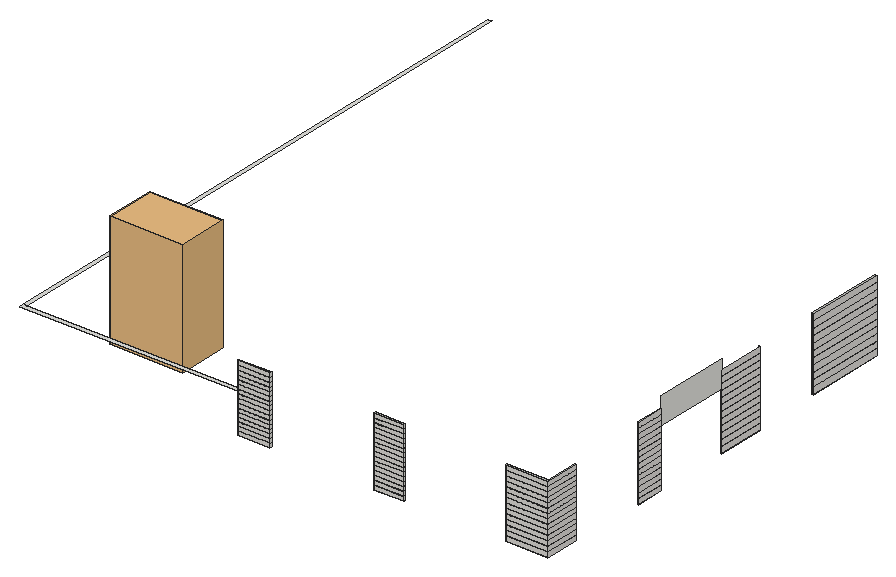
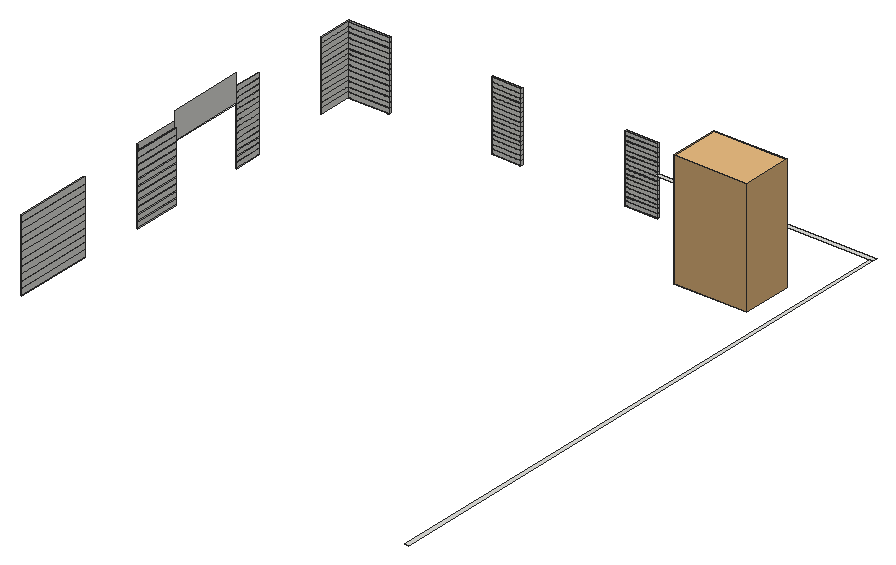
# SketchUp Ruby script. Lengths in inches.
U = 1.inch
M = Sketchup.active_model
def pt(a) = Geom::Point3d.new(a.map { |v| v * U })
def face(e, loops, mat)
  f = e.add_face(loops[0].map { |a| pt(a) })
  loops[1..].each { |l| e.add_face(l.map { |a| pt(a) }).erase! }
  f.material = f.back_material = mat if mat
  f
end
# faces: each face lists its corners as indices into pts; further lists are holes
def faces(e, pts, list, mat = nil) = list.each { |f| face(e, (f[0].is_a?(Array) ? f : [f]).map { |l| l.map { |i| pts[i] } }, mat) }
# xy, xz, yz: faces in a plane at the given z, y or x. An outline is a flat list of corners, or four numbers for a rectangle; further outlines are holes
def ring(l) = l.size == 4 ? [[l[0], l[1]], [l[2], l[1]], [l[2], l[3]], [l[0], l[3]]] : l.each_slice(2).to_a
def flat(e, list, mat, &to3) = list.each { |f| face(e, (f[0].is_a?(Array) ? f : [f]).map { |l| ring(l).map { |u, v| to3.(u, v) } }, mat) }
def xy(e, z, list, mat = nil) = flat(e, list, mat) { |x, y| [x, y, z] }
def xz(e, y, list, mat = nil) = flat(e, list, mat) { |x, z| [x, y, z] }
def yz(e, x, list, mat = nil) = flat(e, list, mat) { |y, z| [x, y, z] }
def lines(e, pts, list) = list.each { |a, b| e.add_line(pt(pts[a]), pt(pts[b])) }
# prism: a flat outline (further loops are holes) pulled along v
def prism(e, loops, v, mat = nil)
  f = face(e, loops, mat); d = Geom::Vector3d.new(v.map { |x| x * U })
  f.pushpull(f.normal.samedirection?(d) ? d.length : -d.length)
end
def box(e, o, s, mat = nil) = prism(e, [[o, [o[0] + s[0], o[1], o[2]], [o[0] + s[0], o[1] + s[1], o[2]], [o[0], o[1] + s[1], o[2]]]], [0, 0, s[2]], mat)
def at(x, y, z, deg = 0) = Geom::Transformation.translation(pt([x, y, z])) * Geom::Transformation.rotation(ORIGIN, Z_AXIS, deg.degrees)
def axes(o, x, y, z) = Geom::Transformation.new([*x, 0, *y, 0, *z, 0, *pt(o).to_a, 1])
def part(name) = M.definitions.add(name)
# library, detail: a bought-in or finely detailed component or shape, given as its bounding box
def library(name, o, s) = part(name).tap { |d| box(d.entities, o, s) }
def detail(e, o, s) = box(e.add_group.entities, o, s)
def put(e, d, t, mat = nil) = e.add_instance(d, t).tap { |i| i.material = mat if mat }
def group(e, t, mat = nil) = e.add_group.tap { |g| g.transformation = t; g.material = mat if mat }.entities
root = M.entities
M.materials.add("[Terrazzo Tile Accent]").color = [224, 221, 217]
c1 = library("tree1",[53.41,58.5,0],[112.17,77.04,177.25])
xy(root,8.42,[[814.625,263.05,816.1875,305.04]])
xy(root,8.5,[[814.625,423.33,816.875,495.84]])
xy(root,9.0625,[[814.625,263.05,816.1875,305.04]])
xy(root,9.44,[[814.625,423.33,816.875,495.84]])
xy(root,11.69,[[547.16,87.66,593.34,90.47]])
xy(root,11.77,[[750.91,87.66,816.1875,87.66,816.1875,140.66,814.625,140.66,814.625,90.47,750.91,90.47]])
xy(root,11.96,[[547.16,87.66,593.34,90.47]])
xy(root,12.4,[[750.91,87.66,750.91,90.47,814.625,90.47,814.625,140.66,816.1875,140.66,816.1875,87.66]])
xy(root,12.86,[[336.5625,87.66,386.78,90.47]])
xy(root,13.19,[[336.5625,87.66,386.78,90.47]])
xy(root,13.92,[[814.625,599,817.6875,719.91]])
xy(root,14.88,[[814.625,599,817.6875,719.91]])
xy(root,16.54,[[814.625,263.05,816.1875,305.04]])
xy(root,17.1875,[[814.625,263.05,816.1875,305.04]])
xy(root,18.43,[[814.625,423.33,816.875,495.84]])
xy(root,18.44,[[547.16,87.66,593.34,90.47]])
xy(root,18.96,[[547.16,87.66,593.34,90.47]])
xy(root,19.26,[[814.625,423.33,816.875,495.84]])
xy(root,19.42,[[336.5625,87.66,386.78,90.47]])
xy(root,19.51,[[336.5625,87.66,386.78,90.47]])
xy(root,19.58,[[750.91,87.66,816.1875,87.66,816.1875,140.66,814.625,140.66,814.625,90.47,750.91,90.47]])
xy(root,20.09,[[750.91,87.66,750.91,90.47,814.625,90.47,814.625,140.66,816.1875,140.66,816.1875,87.66]])
xy(root,24.04,[[814.625,599,817.6875,719.91]])
xy(root,24.67,[[814.625,263.05,816.1875,305.04]])
xy(root,25.01,[[814.625,599,817.6875,719.91]])
xy(root,25.3125,[[814.625,263.05,816.1875,305.04]])
xy(root,25.44,[[547.16,87.66,593.34,90.47]])
xy(root,25.73,[[336.5625,87.66,386.78,90.47]])
xy(root,25.84,[[547.16,87.66,593.34,90.47]])
xy(root,25.88,[[336.5625,87.66,386.78,90.47]])
xy(root,27.27,[[750.91,87.66,816.1875,87.66,816.1875,140.66,814.625,140.66,814.625,90.47,750.91,90.47]])
xy(root,27.71,[[750.91,87.66,750.91,90.47,814.625,90.47,814.625,140.66,816.1875,140.66,816.1875,87.66]])
xy(root,28.25,[[814.625,423.33,816.875,495.84]])
xy(root,28.94,[[814.625,423.33,816.875,495.84]])
xy(root,32.11,[[336.5625,87.66,386.78,90.47]])
xy(root,32.26,[[336.5625,87.66,386.78,90.47]])
xy(root,32.32,[[547.16,87.66,593.34,90.47]])
xy(root,32.4,[[547.16,87.66,593.34,90.47]])
xy(root,32.79,[[814.625,263.05,816.1875,305.04]])
xy(root,33.4375,[[814.625,263.05,816.1875,305.04]])
xy(root,34.17,[[814.625,599,817.6875,719.91]])
xy(root,34.9,[[750.91,87.66,816.1875,87.66,816.1875,140.66,814.625,140.66,814.625,90.47,750.91,90.47]])
xy(root,35.13,[[814.625,599,817.6875,719.91]])
xy(root,35.34,[[750.91,87.66,750.91,90.47,814.625,90.47,814.625,140.66,816.1875,140.66,816.1875,87.66]])
xy(root,37.93,[[814.625,423.33,816.875,495.84]])
xy(root,38.48,[[336.5625,87.66,386.78,90.47]])
xy(root,38.63,[[336.5625,87.66,386.78,90.47],[814.625,423.33,816.875,495.84]])
xy(root,38.88,[[547.16,87.66,593.34,90.47]])
xy(root,38.9,[[547.16,87.66,593.34,90.47]])
xy(root,40.92,[[814.625,263.05,816.1875,305.04]])
xy(root,41.5625,[[814.625,263.05,816.1875,305.04]])
xy(root,42.52,[[750.91,87.66,816.1875,87.66,816.1875,140.66,814.625,140.66,814.625,90.47,750.91,90.47]])
xy(root,42.96,[[750.91,87.66,750.91,90.47,814.625,90.47,814.625,140.66,816.1875,140.66,816.1875,87.66]])
xy(root,44.29,[[814.625,599,817.6875,719.91]])
xy(root,44.86,[[336.5625,87.66,386.78,90.47]])
xy(root,44.94,[[336.5625,87.66,386.78,90.47]])
xy(root,45.26,[[814.625,599,817.6875,719.91]])
xy(root,45.38,[[547.16,87.66,593.34,90.47]])
xy(root,45.46,[[547.16,87.66,593.34,90.47]])
xy(root,47.62,[[814.625,423.33,816.875,495.84]])
xy(root,48.32,[[814.625,423.33,816.875,495.84]])
xy(root,49.04,[[814.625,263.05,816.1875,305.04]])
xy(root,49.6875,[[814.625,263.05,816.1875,305.04]])
xy(root,50.15,[[750.91,87.66,816.1875,87.66,816.1875,140.66,814.625,140.66,814.625,90.47,750.91,90.47]])
xy(root,50.59,[[750.91,87.66,750.91,90.47,814.625,90.47,814.625,140.66,816.1875,140.66,816.1875,87.66]])
xy(root,51.17,[[336.5625,87.66,386.78,90.47]])
xy(root,51.32,[[336.5625,87.66,386.78,90.47]])
xy(root,51.94,[[547.16,87.66,593.34,90.47]])
xy(root,52.03,[[547.16,87.66,593.34,90.47]])
xy(root,54.42,[[814.625,599,817.6875,719.91]])
xy(root,55.38,[[814.625,599,817.6875,719.91]])
xy(root,57.17,[[814.625,263.05,816.1875,305.04]])
xy(root,57.31,[[814.625,423.33,816.875,495.84]])
xy(root,57.54,[[336.5625,87.66,386.78,90.47]])
xy(root,57.77,[[750.91,87.66,816.1875,87.66,816.1875,140.66,814.625,140.66,814.625,90.47,750.91,90.47]])
xy(root,57.8125,[[814.625,263.05,816.1875,305.04]])
xy(root,57.94,[[336.5625,87.66,386.78,90.47]])
xy(root,58.01,[[814.625,423.33,816.875,495.84]])
xy(root,58.15,[[750.91,87.66,750.91,90.47,814.625,90.47,814.625,140.66,816.1875,140.66,816.1875,87.66]])
xy(root,58.5,[[547.16,87.66,593.34,90.47]])
xy(root,58.58,[[547.16,87.66,593.34,90.47]])
xy(root,64.17,[[336.5625,87.66,386.78,90.47]])
xy(root,64.54,[[814.625,599,817.6875,719.91]])
xy(root,64.71,[[336.5625,87.66,386.78,90.47]])
xy(root,65.06,[[547.16,87.66,593.34,90.47]])
xy(root,65.14,[[547.16,87.66,593.34,90.47]])
xy(root,65.29,[[814.625,263.05,816.1875,305.04]])
xy(root,65.33,[[750.91,87.66,816.1875,87.66,816.1875,140.66,814.625,140.66,814.625,90.47,750.91,90.47]])
xy(root,65.51,[[814.625,599,817.6875,719.91]])
xy(root,65.59,[[750.91,87.66,750.91,90.47,814.625,90.47,814.625,140.66,816.1875,140.66,816.1875,87.66]])
xy(root,65.9375,[[814.625,263.05,816.1875,305.04]])
xy(root,67,[[814.625,423.33,816.875,495.84]])
xy(root,67.69,[[814.625,423.33,816.875,495.84]])
xy(root,70.93,[[336.5625,87.66,386.78,90.47]])
xy(root,71.08,[[336.5625,87.66,386.78,90.47]])
xy(root,71.62,[[547.16,87.66,593.34,90.47]])
xy(root,71.77,[[547.16,87.66,593.34,90.47]])
xy(root,72.77,[[750.91,87.66,816.1875,87.66,816.1875,140.66,814.625,140.66,814.625,90.47,750.91,90.47]])
xy(root,73.03,[[750.91,87.66,750.91,90.47,814.625,90.47,814.625,140.66,816.1875,140.66,816.1875,87.66]])
xy(root,73.42,[[814.625,263.05,816.1875,305.04]])
xy(root,74.0625,[[814.625,263.05,816.1875,305.04]])
xy(root,74.67,[[814.625,599,817.6875,719.91]])
xy(root,75.63,[[814.625,599,817.6875,719.91]])
xy(root,76.68,[[814.625,423.33,816.875,495.84]])
xy(root,77.31,[[336.5625,87.66,386.78,90.47]])
xy(root,77.38,[[814.625,423.33,816.875,495.84]])
xy(root,77.52,[[336.5625,87.66,386.78,90.47]])
xy(root,78.25,[[547.16,87.66,593.34,90.47]])
xy(root,78.32,[[547.16,87.66,593.34,90.47]])
xy(root,80.21,[[750.91,87.66,816.1875,87.66,816.1875,140.66,814.625,140.66,814.625,90.47,750.91,90.47]])
xy(root,80.49,[[750.91,87.66,750.91,90.47,814.625,90.47,814.625,140.66,816.1875,140.66,816.1875,87.66]])
xy(root,81.54,[[814.625,263.05,816.1875,305.04]])
xy(root,82.1875,[[814.625,263.05,816.1875,305.04]])
xy(root,83.74,[[336.5625,87.66,386.78,90.47]])
xy(root,84.02,[[336.5625,87.66,386.78,90.47]])
xy(root,84.79,[[814.625,599,817.6875,719.91]])
xy(root,84.8,[[547.16,87.66,593.34,90.47]])
xy(root,84.95,[[547.16,87.66,593.34,90.47]])
xy(root,85.76,[[814.625,599,817.6875,719.91]])
xy(root,86.37,[[814.625,423.33,816.875,495.84]])
xy(root,87.07,[[814.625,423.33,816.875,495.84]])
xy(root,87.67,[[750.91,87.66,816.1875,87.66,816.1875,140.66,814.625,140.66,814.625,90.47,750.91,90.47]])
xy(root,87.99,[[750.91,87.66,750.91,90.47,814.625,90.47,814.625,140.66,816.1875,140.66,816.1875,87.66]])
xy(root,89.67,[[814.625,263.05,816.1875,305.04]])
xy(root,90.24,[[336.5625,87.66,386.78,90.47]])
xy(root,90.3125,[[814.625,263.05,816.1875,305.04]])
xy(root,90.52,[[336.5625,87.66,386.78,90.47]])
xy(root,91.42,[[547.16,87.66,593.34,90.47]])
xy(root,91.57,[[547.16,87.66,593.34,90.47]])
xy(root,94.92,[[814.625,599,817.6875,719.91]])
xy(root,95.17,[[750.91,87.66,816.1875,87.66,816.1875,140.66,814.625,140.66,814.625,90.47,750.91,90.47]])
xy(root,95.43,[[750.91,87.66,750.91,90.47,814.625,90.47,814.625,140.66,816.1875,140.66,816.1875,87.66]])
xy(root,95.88,[[814.625,599,817.6875,719.91]])
xy(root,96.06,[[814.625,423.33,816.875,495.84]])
xy(root,96.74,[[336.5625,87.66,386.78,90.47]])
xy(root,96.76,[[814.625,423.33,816.875,495.84]])
xy(root,96.96,[[336.5625,87.66,386.78,90.47]])
xy(root,97.79,[[814.625,263.05,816.1875,305.04]])
xy(root,98.05,[[547.16,87.66,593.34,90.47]])
xy(root,98.2,[[547.16,87.66,593.34,90.47]])
xy(root,98.4375,[[814.625,263.05,816.1875,305.04],[814.625,305.04,816.1875,423.04],[814.625,423.04,816.1875,423.33]])
xy(root,102.61,[[750.91,87.66,816.1875,87.66,816.1875,140.66,814.625,140.66,814.625,90.47,750.91,90.47]])
xy(root,102.86,[[750.91,87.66,750.91,90.47,814.625,90.47,814.625,140.66,816.1875,140.66,816.1875,87.66]])
xy(root,103.18,[[336.5625,87.66,386.78,90.47]])
xy(root,103.71,[[336.5625,87.66,386.78,90.47]])
xy(root,104.67,[[547.16,87.66,593.34,90.47]])
xy(root,104.88,[[547.16,87.66,593.34,90.47]])
xy(root,105.04,[[814.625,599,817.6875,719.91]])
xy(root,105.75,[[814.625,423.33,816.875,495.84]])
xy(root,105.92,[[814.625,263.05,816.1875,305.04]])
xy(root,106.01,[[814.625,599,817.6875,719.91]])
xy(root,106.44,[[814.625,423.33,816.875,495.84]])
xy(root,106.5625,[[814.625,263.05,816.1875,305.04]])
xy(root,109.93,[[336.5625,87.66,386.78,90.47]])
xy(root,110.05,[[750.91,87.66,816.1875,87.66,816.1875,140.66,814.625,140.66,814.625,90.47,750.91,90.47]])
xy(root,110.36,[[750.91,87.66,750.91,90.47,814.625,90.47,814.625,140.66,816.1875,140.66,816.1875,87.66]])
xy(root,110.46,[[336.5625,87.66,386.78,90.47]])
xy(root,111.36,[[547.16,87.66,593.34,90.47]])
xy(root,111.7,[[547.16,87.66,593.34,90.47]])
xy(root,114.04,[[814.625,263.05,816.1875,305.04]])
xy(root,114.6875,[[814.625,263.05,816.1875,305.04]])
xy(root,115.17,[[814.625,599,817.6875,719.91]])
xy(root,115.43,[[814.625,423.33,816.875,495.84]])
xy(root,116.13,[[814.625,423.33,816.875,495.84],[814.625,599,817.6875,719.91]])
xz(root,87.66,[[547.16,11.96,593.34,18.44],[750.91,12.4,816.1875,19.58],[336.5625,13.19,386.78,19.42],[547.16,18.96,593.34,25.44],[336.5625,19.51,386.78,25.73],
  [750.91,20.09,816.1875,27.27],[547.16,25.84,593.34,32.32],[336.5625,25.88,386.78,32.11],[750.91,27.71,816.1875,34.9],[336.5625,32.26,386.78,38.48],
  [547.16,32.4,593.34,38.88],[750.91,35.34,816.1875,42.52],[336.5625,38.63,386.78,44.86],[547.16,38.9,593.34,45.38],[750.91,42.96,816.1875,50.15],
  [336.5625,44.94,386.78,51.17],[547.16,45.46,593.34,51.94],[750.91,50.59,816.1875,57.77],[336.5625,51.32,386.78,57.54],[547.16,52.03,593.34,58.5],
  [336.5625,57.94,386.78,64.17],[750.91,58.15,816.1875,65.33],[547.16,58.58,593.34,65.06],[336.5625,64.71,386.78,70.93],[547.16,65.14,593.34,71.62],
  [750.91,65.59,816.1875,72.77],[336.5625,71.08,386.78,77.31],[547.16,71.77,593.34,78.25],[750.91,73.03,816.1875,80.21],[336.5625,77.52,386.78,83.74],
  [547.16,78.32,593.34,84.8],[750.91,80.49,816.1875,87.67],[336.5625,84.02,386.78,90.24],[547.16,84.95,593.34,91.42],[750.91,87.99,816.1875,95.17],
  [336.5625,90.52,386.78,96.74],[547.16,91.57,593.34,98.05],[750.91,95.43,816.1875,102.61],[336.5625,96.96,386.78,103.18],[547.16,98.2,593.34,104.67],
  [750.91,102.86,816.1875,110.05],[336.5625,103.71,386.78,109.93],[547.16,104.88,593.34,111.36],[750.91,110.36,816.1875,117.55],[336.5625,110.46,386.78,116.68],
  [547.16,111.7,593.34,118.17]],"[Terrazzo Tile Accent]")
xz(root,90.47,[[547.16,11.69,593.34,11.96],[750.91,11.77,814.625,12.4],[547.16,11.96,593.34,18.44],[750.91,12.4,814.625,19.58],[336.5625,12.86,386.78,13.19],
  [336.5625,13.19,386.78,19.42],[547.16,18.44,593.34,18.96],[547.16,18.96,593.34,25.44],[336.5625,19.42,386.78,19.51],[336.5625,19.51,386.78,25.73],
  [750.91,19.58,814.625,20.09],[750.91,20.09,814.625,27.27],[547.16,25.44,593.34,25.84],[336.5625,25.73,386.78,25.88],[547.16,25.84,593.34,32.32],
  [336.5625,25.88,386.78,32.11],[750.91,27.27,814.625,27.71],[750.91,27.71,814.625,34.9],[336.5625,32.11,386.78,32.26],[336.5625,32.26,386.78,38.48],
  [547.16,32.32,593.34,32.4],[547.16,32.4,593.34,38.88],[750.91,34.9,814.625,35.34],[750.91,35.34,814.625,42.52],[336.5625,38.48,386.78,38.63],
  [336.5625,38.63,386.78,44.86],[547.16,38.88,593.34,38.9],[547.16,38.9,593.34,45.38],[750.91,42.52,814.625,42.96],[750.91,42.96,814.625,50.15],
  [336.5625,44.86,386.78,44.94],[336.5625,44.94,386.78,51.17],[547.16,45.38,593.34,45.46],[547.16,45.46,593.34,51.94],[750.91,50.15,814.625,50.59],
  [750.91,50.59,814.625,57.77],[336.5625,51.17,386.78,51.32],[336.5625,51.32,386.78,57.54],[547.16,51.94,593.34,52.03],[547.16,52.03,593.34,58.5],
  [336.5625,57.54,386.78,57.94],[750.91,57.77,814.625,58.15],[336.5625,57.94,386.78,64.17],[750.91,58.15,814.625,65.33],[547.16,58.5,593.34,58.58],
  [547.16,58.58,593.34,65.06],[336.5625,64.17,386.78,64.71],[336.5625,64.71,386.78,70.93],[547.16,65.06,593.34,65.14],[547.16,65.14,593.34,71.62],
  [750.91,65.33,814.625,65.59],[750.91,65.59,814.625,72.77],[336.5625,70.93,386.78,71.08],[336.5625,71.08,386.78,77.31],[547.16,71.62,593.34,71.77],
  [547.16,71.77,593.34,78.25],[750.91,72.77,814.625,73.03],[750.91,73.03,814.625,80.21],[336.5625,77.31,386.78,77.52],[336.5625,77.52,386.78,83.74],
  [547.16,78.25,593.34,78.32],[547.16,78.32,593.34,84.8],[750.91,80.21,814.625,80.49],[750.91,80.49,814.625,87.67],[336.5625,83.74,386.78,84.02],
  [336.5625,84.02,386.78,90.24],[547.16,84.8,593.34,84.95],[547.16,84.95,593.34,91.42],[750.91,87.67,814.625,87.99],[750.91,87.99,814.625,95.17],
  [336.5625,90.24,386.78,90.52],[336.5625,90.52,386.78,96.74],[547.16,91.42,593.34,91.57],[547.16,91.57,593.34,98.05],[750.91,95.17,814.625,95.43],
  [750.91,95.43,814.625,102.61],[336.5625,96.74,386.78,96.96],[336.5625,96.96,386.78,103.18],[547.16,98.05,593.34,98.2],[547.16,98.2,593.34,104.67],
  [750.91,102.61,814.625,102.86],[750.91,102.86,814.625,110.05],[336.5625,103.18,386.78,103.71],[336.5625,103.71,386.78,109.93],[547.16,104.67,593.34,104.88],
  [547.16,104.88,593.34,111.36],[336.5625,109.93,386.78,110.46],[750.91,110.05,814.625,110.36],[750.91,110.36,814.625,117.55],[336.5625,110.46,386.78,116.68],
  [547.16,111.36,593.34,111.7],[547.16,111.7,593.34,118.17]])
xz(root,140.66,[[814.625,12.4,816.1875,19.58],[814.625,20.09,816.1875,27.27],[814.625,27.71,816.1875,34.9],[814.625,35.34,816.1875,42.52],[814.625,42.96,816.1875,50.15],
  [814.625,50.59,816.1875,57.77],[814.625,58.15,816.1875,65.33],[814.625,65.59,816.1875,72.77],[814.625,73.03,816.1875,80.21],[814.625,80.49,816.1875,87.67],
  [814.625,87.99,816.1875,95.17],[814.625,95.43,816.1875,102.61],[814.625,102.86,816.1875,110.05],[814.625,110.36,816.1875,117.55]])
xz(root,263.05,[[814.625,9.0625,816.1875,16.54],[814.625,17.1875,816.1875,24.67],[814.625,25.3125,816.1875,32.79],[814.625,33.4375,816.1875,40.92],[814.625,41.5625,816.1875,49.04],
  [814.625,49.6875,816.1875,57.17],[814.625,57.8125,816.1875,65.29],[814.625,65.9375,816.1875,73.42],[814.625,74.0625,816.1875,81.54],[814.625,82.1875,816.1875,89.67],
  [814.625,90.3125,816.1875,97.79],[814.625,98.4375,816.1875,105.92],[814.625,106.5625,816.1875,114.04],[814.625,114.6875,816.1875,122.17]])
xz(root,305.04,[[814.625,9.0625,816.1875,16.54],[814.625,17.1875,816.1875,24.67],[814.625,25.3125,816.1875,32.79],[814.625,33.4375,816.1875,40.92],[814.625,41.5625,816.1875,49.04],
  [814.625,49.6875,816.1875,57.17],[814.625,57.8125,816.1875,65.29],[814.625,65.9375,816.1875,73.42],[814.625,74.0625,816.1875,81.54],[814.625,82.1875,816.1875,89.67],
  [814.625,90.3125,816.1875,97.79],[814.625,98.4375,816.1875,105.92],[814.625,105.92,816.1875,106.5625],[814.625,106.5625,816.1875,114.04],[814.625,114.04,816.1875,114.6875],
  [814.625,114.6875,816.1875,122.17]])
xz(root,423.33,[[814.625,9.44,816.875,18.43],[814.625,19.26,816.875,28.25],[814.625,28.94,816.875,37.93],[814.625,38.63,816.875,47.62],[814.625,48.32,816.875,57.31],
  [814.625,58.01,816.875,67],[814.625,67.69,816.875,76.68],[814.625,77.38,816.875,86.37],[814.625,87.07,816.875,96.06],[814.625,96.76,816.875,96.76,816.875,105.75,816.1875,105.75,816.1875,98.4375,814.625,98.4375],
  [814.625,98.4375,816.1875,105.75],[814.625,105.75,816.1875,106.44],[814.625,106.44,816.1875,115.43],[816.1875,106.44,816.875,115.43],[814.625,115.43,816.1875,116.13],
  [816.1875,116.13,816.875,125.12]])
xz(root,495.84,[[814.625,19.26,816.875,28.25],[814.625,28.94,816.875,37.93],[814.625,38.63,816.875,47.62],[814.625,48.32,816.875,57.31],[814.625,58.01,816.875,67],
  [814.625,67.69,816.875,76.68],[814.625,77.38,816.875,86.37],[814.625,87.07,816.875,96.06],[814.625,96.76,816.875,105.75],[814.625,106.44,816.875,115.43],
  [814.625,116.13,816.875,125.12]])
xz(root,599,[[814.625,14.88,817.6875,24.04],[814.625,25.01,817.6875,34.17],[814.625,35.13,817.6875,44.29],[814.625,45.26,817.6875,54.42],[814.625,55.38,817.6875,64.54],
  [814.625,65.51,817.6875,74.67],[814.625,75.63,817.6875,84.79],[814.625,85.76,817.6875,94.92],[814.625,95.88,817.6875,105.04],[814.625,106.01,817.6875,115.17],
  [814.625,116.13,817.6875,125.29]])
xz(root,719.91,[[814.625,14.88,817.6875,24.04],[814.625,25.01,817.6875,34.17],[814.625,35.13,817.6875,44.29],[814.625,45.26,817.6875,54.42],[814.625,55.38,817.6875,64.54],
  [814.625,65.51,817.6875,74.67],[814.625,75.63,817.6875,84.79],[814.625,85.76,817.6875,94.92],[814.625,95.88,817.6875,105.04],[814.625,106.01,817.6875,115.17],
  [814.625,116.13,817.6875,125.29]])
yz(root,336.5625,[[87.66,13.19,90.47,19.42],[87.66,19.51,90.47,25.73],[87.66,25.88,90.47,32.11],[87.66,32.26,90.47,38.48],[87.66,38.63,90.47,44.86],
  [87.66,44.94,90.47,51.17],[87.66,51.32,90.47,57.54],[87.66,57.94,90.47,64.17],[87.66,64.71,90.47,70.93],[87.66,71.08,90.47,77.31],
  [87.66,77.52,90.47,83.74],[87.66,84.02,90.47,90.24],[87.66,90.52,90.47,96.74],[87.66,96.96,90.47,103.18],[87.66,103.71,90.47,109.93],
  [87.66,110.46,90.47,116.68]])
yz(root,386.78,[[87.66,13.19,90.47,19.42],[87.66,19.51,90.47,25.73],[87.66,25.88,90.47,32.11],[87.66,32.26,90.47,38.48],[87.66,38.63,90.47,44.86],
  [87.66,44.94,90.47,51.17],[87.66,51.32,90.47,57.54],[87.66,57.94,90.47,64.17],[87.66,64.71,90.47,70.93],[87.66,71.08,90.47,77.31],
  [87.66,77.52,90.47,83.74],[87.66,84.02,90.47,90.24],[87.66,90.52,90.47,96.74],[87.66,96.96,90.47,103.18],[87.66,103.71,90.47,109.93],
  [87.66,110.46,90.47,116.68]])
yz(root,547.16,[[87.66,11.96,90.47,18.44],[87.66,18.96,90.47,25.44],[87.66,25.84,90.47,32.32],[87.66,32.4,90.47,38.88],[87.66,38.9,90.47,45.38],
  [87.66,45.46,90.47,51.94],[87.66,52.03,90.47,58.5],[87.66,58.58,90.47,65.06],[87.66,65.14,90.47,71.62],[87.66,71.77,90.47,78.25],
  [87.66,78.32,90.47,84.8],[87.66,84.95,90.47,91.42],[87.66,91.57,90.47,98.05],[87.66,98.2,90.47,104.67],[87.66,104.88,90.47,111.36],
  [87.66,111.7,90.47,118.17]])
yz(root,593.34,[[87.66,11.96,90.47,18.44],[87.66,18.96,90.47,25.44],[87.66,25.84,90.47,32.32],[87.66,32.4,90.47,38.88],[87.66,38.9,90.47,45.38],
  [87.66,45.46,90.47,51.94],[87.66,52.03,90.47,58.5],[87.66,58.58,90.47,65.06],[87.66,65.14,90.47,71.62],[87.66,71.77,90.47,78.25],
  [87.66,78.32,90.47,84.8],[87.66,84.95,90.47,91.42],[87.66,91.57,90.47,98.05],[87.66,98.2,90.47,104.67],[87.66,104.88,90.47,111.36],
  [87.66,111.7,90.47,118.17]])
yz(root,750.91,[[87.66,12.4,90.47,19.58],[87.66,20.09,90.47,27.27],[87.66,27.71,90.47,34.9],[87.66,35.34,90.47,42.52],[87.66,42.96,90.47,50.15],
  [87.66,50.59,90.47,57.77],[87.66,58.15,90.47,65.33],[87.66,65.59,90.47,72.77],[87.66,73.03,90.47,80.21],[87.66,80.49,90.47,87.67],
  [87.66,87.99,90.47,95.17],[87.66,95.43,90.47,102.61],[87.66,102.86,90.47,110.05],[87.66,110.36,90.47,117.55]])
yz(root,814.625,[[263.05,8.42,305.04,9.0625],[423.33,8.5,495.84,9.44],[263.05,9.0625,305.04,16.54],[423.33,9.44,495.84,18.43],[90.47,12.4,140.66,19.58],
  [599,14.88,719.91,24.04],[263.05,16.54,305.04,17.1875],[263.05,17.1875,305.04,24.67],[423.33,18.43,495.84,19.26],[423.33,19.26,495.84,28.25],
  [90.47,20.09,140.66,27.27],[263.05,24.67,305.04,25.3125],[599,25.01,719.91,34.17],[263.05,25.3125,305.04,32.79],[90.47,27.71,140.66,34.9],
  [423.33,28.25,495.84,28.94],[423.33,28.94,495.84,37.93],[263.05,32.79,305.04,33.4375],[263.05,33.4375,305.04,40.92],[599,35.13,719.91,44.29],
  [90.47,35.34,140.66,42.52],[423.33,37.93,495.84,38.63],[423.33,38.63,495.84,47.62],[263.05,40.92,305.04,41.5625],[263.05,41.5625,305.04,49.04],
  [90.47,42.96,140.66,50.15],[599,45.26,719.91,54.42],[423.33,47.62,495.84,48.32],[423.33,48.32,495.84,57.31],[263.05,49.04,305.04,49.6875],
  [263.05,49.6875,305.04,57.17],[90.47,50.59,140.66,57.77],[599,55.38,719.91,64.54],[263.05,57.17,305.04,57.8125],[423.33,57.31,495.84,58.01],
  [263.05,57.8125,305.04,65.29],[423.33,58.01,495.84,67],[90.47,58.15,140.66,65.33],[263.05,65.29,305.04,65.9375],[599,65.51,719.91,74.67],
  [90.47,65.59,140.66,72.77],[263.05,65.9375,305.04,73.42],[423.33,67,495.84,67.69],[423.33,67.69,495.84,76.68],[90.47,73.03,140.66,80.21],
  [263.05,73.42,305.04,74.0625],[263.05,74.0625,305.04,81.54],[599,75.63,719.91,84.79],[423.33,76.68,495.84,77.38],[423.33,77.38,495.84,86.37],
  [90.47,80.49,140.66,87.67],[263.05,81.54,305.04,82.1875],[263.05,82.1875,305.04,89.67],[599,85.76,719.91,94.92],[423.33,86.37,495.84,87.07],
  [423.33,87.07,495.84,96.06],[90.47,87.99,140.66,95.17],[263.05,89.67,305.04,90.3125],[263.05,90.3125,305.04,97.79],[90.47,95.43,140.66,102.61],
  [599,95.88,719.91,105.04],[423.33,96.06,495.84,96.76],[423.33,96.76,495.84,105.75],[263.05,97.79,305.04,98.4375],[263.05,98.4375,305.04,105.92],
  [90.47,102.86,140.66,110.05],[423.33,105.75,495.84,106.44],[263.05,105.92,305.04,106.5625],[599,106.01,719.91,115.17],[423.33,106.44,495.84,115.43],
  [263.05,106.5625,305.04,114.04],[90.47,110.36,140.66,117.55],[263.05,114.04,305.04,114.6875],[263.05,114.6875,305.04,122.17],[423.33,115.43,495.84,116.13],
  [599,116.13,719.91,125.29]])
yz(root,816.1875,[[305.04,98.4375,423.33,140.0625]])
yz(root,816.1875,[[263.05,9.0625,305.04,16.54],[87.66,12.4,140.66,19.58],[263.05,17.1875,305.04,24.67],[87.66,20.09,140.66,27.27],[263.05,25.3125,305.04,32.79],
  [87.66,27.71,140.66,34.9],[263.05,33.4375,305.04,40.92],[87.66,35.34,140.66,42.52],[263.05,41.5625,305.04,49.04],[87.66,42.96,140.66,50.15],
  [263.05,49.6875,305.04,57.17],[87.66,50.59,140.66,57.77],[263.05,57.8125,305.04,65.29],[87.66,58.15,140.66,65.33],[87.66,65.59,140.66,72.77],
  [263.05,65.9375,305.04,73.42],[87.66,73.03,140.66,80.21],[263.05,74.0625,305.04,81.54],[87.66,80.49,140.66,87.67],[263.05,82.1875,305.04,89.67],
  [87.66,87.99,140.66,95.17],[263.05,90.3125,305.04,97.79],[87.66,95.43,140.66,102.61],[263.05,98.4375,305.04,105.92],[87.66,102.86,140.66,110.05],
  [263.05,106.5625,305.04,114.04],[87.66,110.36,140.66,117.55],[263.05,114.6875,305.04,122.17]],"[Terrazzo Tile Accent]")
yz(root,816.875,[[423.33,9.44,495.84,18.43],[423.33,19.26,495.84,28.25],[423.33,28.94,495.84,37.93],[423.33,38.63,495.84,47.62],[423.33,48.32,495.84,57.31],
  [423.33,58.01,495.84,67],[423.33,67.69,495.84,76.68],[423.33,77.38,495.84,86.37],[423.33,87.07,495.84,96.06],[423.33,96.76,495.84,105.75],
  [423.33,106.44,495.84,115.43],[423.33,116.13,495.84,125.12]],"[Terrazzo Tile Accent]")
yz(root,817.6875,[[599,14.88,719.91,24.04],[599,25.01,719.91,34.17],[599,35.13,719.91,44.29],[599,45.26,719.91,54.42],[599,55.38,719.91,64.54],
  [599,65.51,719.91,74.67],[599,75.63,719.91,84.79],[599,85.76,719.91,94.92],[599,95.88,719.91,105.04],[599,106.01,719.91,115.17],
  [599,116.13,719.91,125.29]],"[Terrazzo Tile Accent]")
p = [[336.43,90.47,74],[336.43,87.66,74],[0.75,87.66,73.42],[0.75,94.42,73.42],[6.1,94.42,73.43],[336.43,94.42,74],
  [6.1,990.97,73.43],[0.75,990.97,73.42]]
faces(root,p,[[0,1,2,3,4,5],[3,4,6,7]])
put(root,c1,at(39.21,87.66,27.53))
